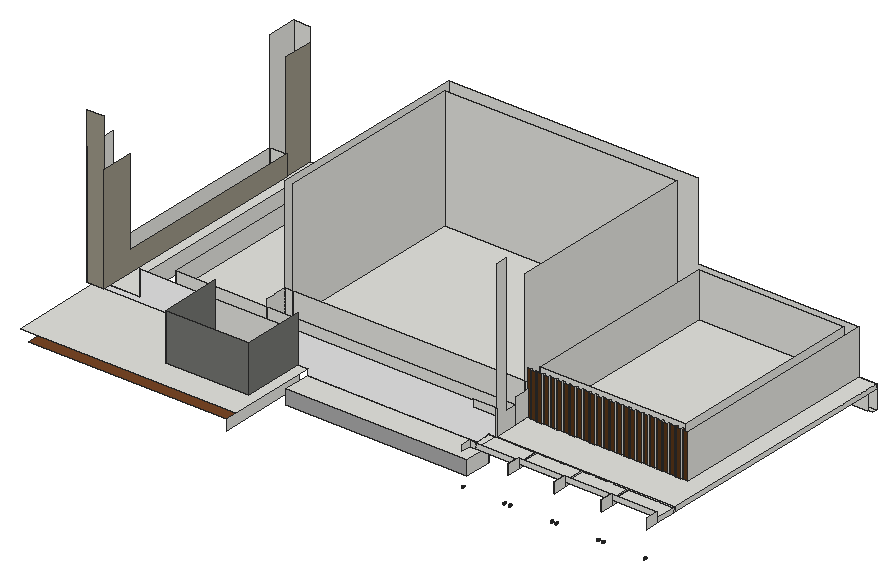
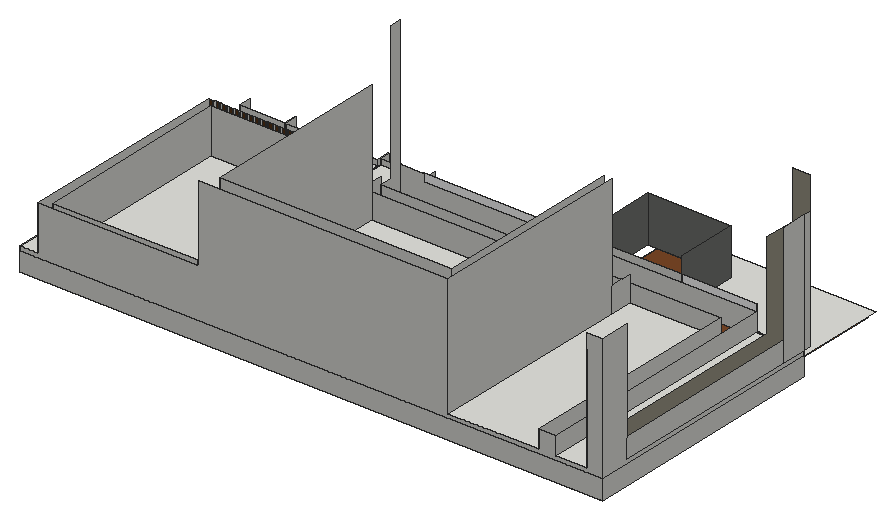
# SketchUp Ruby script. Lengths in inches.
U = 1.inch
M = Sketchup.active_model
def pt(a) = Geom::Point3d.new(a.map { |v| v * U })
def face(e, loops, mat)
  f = e.add_face(loops[0].map { |a| pt(a) })
  loops[1..].each { |l| e.add_face(l.map { |a| pt(a) }).erase! }
  f.material = f.back_material = mat if mat
  f
end
# faces: each face lists its corners as indices into pts; further lists are holes
def faces(e, pts, list, mat = nil) = list.each { |f| face(e, (f[0].is_a?(Array) ? f : [f]).map { |l| l.map { |i| pts[i] } }, mat) }
# xy, xz, yz: faces in a plane at the given z, y or x. An outline is a flat list of corners, or four numbers for a rectangle; further outlines are holes
def ring(l) = l.size == 4 ? [[l[0], l[1]], [l[2], l[1]], [l[2], l[3]], [l[0], l[3]]] : l.each_slice(2).to_a
def flat(e, list, mat, &to3) = list.each { |f| face(e, (f[0].is_a?(Array) ? f : [f]).map { |l| ring(l).map { |u, v| to3.(u, v) } }, mat) }
def xy(e, z, list, mat = nil) = flat(e, list, mat) { |x, y| [x, y, z] }
def xz(e, y, list, mat = nil) = flat(e, list, mat) { |x, z| [x, y, z] }
def yz(e, x, list, mat = nil) = flat(e, list, mat) { |y, z| [x, y, z] }
def lines(e, pts, list) = list.each { |a, b| e.add_line(pt(pts[a]), pt(pts[b])) }
# prism: a flat outline (further loops are holes) pulled along v
def prism(e, loops, v, mat = nil)
  f = face(e, loops, mat); d = Geom::Vector3d.new(v.map { |x| x * U })
  f.pushpull(f.normal.samedirection?(d) ? d.length : -d.length)
end
def box(e, o, s, mat = nil) = prism(e, [[o, [o[0] + s[0], o[1], o[2]], [o[0] + s[0], o[1] + s[1], o[2]], [o[0], o[1] + s[1], o[2]]]], [0, 0, s[2]], mat)
def at(x, y, z, deg = 0) = Geom::Transformation.translation(pt([x, y, z])) * Geom::Transformation.rotation(ORIGIN, Z_AXIS, deg.degrees)
def axes(o, x, y, z) = Geom::Transformation.new([*x, 0, *y, 0, *z, 0, *pt(o).to_a, 1])
def part(name) = M.definitions.add(name)
# library, detail: a bought-in or finely detailed component or shape, given as its bounding box
def library(name, o, s) = part(name).tap { |d| box(d.entities, o, s) }
def detail(e, o, s) = box(e.add_group.entities, o, s)
def put(e, d, t, mat = nil) = e.add_instance(d, t).tap { |i| i.material = mat if mat }
def group(e, t, mat = nil) = e.add_group.tap { |g| g.transformation = t; g.material = mat if mat }.entities
root = M.entities
M.materials.add("[0030_OldLace]").color = [86, 53, 24]
M.materials.add("[0128_White]").color = [255, 255, 255]
M.materials.add("[Color M03]").color = [170, 170, 170]
M.materials.add("[Concrete Tile]").color = [155, 150, 134]
M.materials.add("[Metal Seamed]").color = [116, 117, 113]
M.materials.add("[Wood Veneer 01]").color = [120, 70, 37]
xy(root,95.79,[[2444.05,846.1,2544.33,851.0625]])
xy(root,99.26,[[2381.36,810.97,2608.61,845.35]],"[Wood Veneer 01]")
xy(root,101.375,[[2305.05,845.35,2370.42,846.1],[2112.0625,846.1,2112.0625,1160.85,2840.8125,1160.85,2840.8125,1155.13,2117.78,1155.13,2117.78,851.0625,2305.05,851.0625,2305.05,846.1],[2305.05,846.1,2370.42,851.0625]])
xy(root,101.78,[[2134.72,845.35,2259.6,851.0625]])
xy(root,114.25,[[2123,732.28,2370.42,845.35]],"[Wood Veneer 01]")
xy(root,117.26,[[2381.36,810.97,2608.61,845.35]])
xy(root,125.1875,[[2112.0625,732.28,2381.36,732.28,2381.36,845.35,2369.43,845.35,2369.43,767.72,2265.24,767.72,2265.24,845.35,2112.0625,845.35],[2112.0625,845.35,2381.36,846.1]])
xy(root,131.1875,[[2608.61,814.22,2609.07,844.47],[2609.07,814.22,2617.01,844.47],[2617.01,814.22,2666.66,844.47],[2667.6,817.6,2724.71,844.47],[2725.77,817.6,2782.76,844.47],
  [2784.08,817.6,2840.8125,844.47],[2112.0625,837.03,2132.8125,845.35],[2608.61,844.47,2609.07,845.35],[2609.07,844.47,2617.01,845.35],[2617.01,844.47,2840.8125,846.1],
  [2112.0625,845.35,2132.8125,846.1],[2132.8125,845.35,2170.98,846.1],[2608.61,845.35,2609.07,846.1],[2609.07,845.35,2617.01,846.1],[2112.0625,846.1,2132.8125,877.14],
  [2132.8125,846.1,2170.98,846.1,2170.98,1160.85,2132.1875,1160.85,2132.1875,1122.97,2132.8125,1122.97],[2617.01,846.1,2840.8125,846.1,2840.8125,1160.85,2818.39,1160.85,2818.39,893.65,2812.24,893.65,2812.24,895.71,2810.07,895.71,2810.07,893.65,2803.93,893.65,2803.93,895.71,2801.76,895.71,2801.76,894.34,2795.61,894.34,2795.61,895.71,2793.45,895.71,2793.45,894.34,2787.3,894.34,2787.3,895.71,2785.14,895.71,2785.14,894.34,2778.99,894.34,2778.99,895.71,2776.82,895.71,2776.82,894.34,2770.68,894.34,2770.68,895.71,2768.51,895.71,2768.51,894.34,2762.36,894.34,2762.36,895.71,2760.2,895.71,2760.2,894.34,2754.05,894.34,2754.05,895.71,2751.89,895.71,2751.89,894.34,2745.74,894.34,2745.74,895.71,2743.57,895.71,2743.57,894.34,2737.43,894.34,2737.43,895.71,2735.26,895.71,2735.26,894.34,2729.11,894.34,2729.11,895.71,2726.95,895.71,2726.95,894.34,2720.8,894.34,2720.8,895.71,2718.64,895.71,2718.64,894.34,2712.49,894.34,2712.49,895.71,2710.32,895.71,2710.32,894.34,2704.18,894.34,2704.18,895.71,2702.01,895.71,2702.01,894.34,2695.86,894.34,2695.86,895.71,2693.7,895.71,2693.7,894.34,2687.55,894.34,2687.55,895.71,2685.39,895.71,2685.39,894.34,2679.24,894.34,2679.24,895.71,2677.07,895.71,2677.07,894.34,2670.93,894.34,2670.93,895.71,2668.76,895.71,2668.76,894.34,2662.61,894.34,2662.61,895.71,2660.45,895.71,2660.45,894.34,2654.3,894.34,2654.3,895.71,2652.14,895.71,2652.14,894.34,2645.99,894.34,2645.99,895.71,2643.82,895.71,2643.82,894.34,2637.68,894.34,2637.68,895.71,2635.51,895.71,2635.51,894.34,2629.36,894.34,2629.36,895.71,2627.2,895.71,2627.2,894.34,2621.05,894.34,2621.05,895.71,2617.01,895.71],[2112.0625,877.14,2132.8125,1122.97],[2191.39,877.14,2305.05,1160.85],[2305.05,877.14,2617.01,905.7],
  [2625.48,904.18,2807.17,1152.375],[2314.43,905.7,2604.75,1143.26]])
xz(root,767.72,[[2265.24,125.1875,2369.43,183.3125]],"[Metal Seamed]")
xz(root,799.91,[[2611.43,91.63,2611.73,91.67,2612,91.78,2612.23,91.96,2612.41,92.19,2612.52,92.46,2612.56,92.75,2612.52,93.04,2612.41,93.32,2612.23,93.55,2612,93.73,2611.73,93.84,2611.43,93.88,2611.14,93.84,2610.87,93.73,2610.64,93.55,2610.46,93.32,2610.35,93.04,2610.31,92.75,2610.35,92.46,2610.46,92.19,2610.64,91.96,2610.87,91.78,2611.14,91.67],[2663.62,91.63,2663.91,91.67,2664.18,91.78,2664.42,91.96,2664.6,92.19,2664.71,92.46,2664.75,92.75,2664.71,93.04,2664.6,93.32,2664.42,93.55,2664.18,93.73,2663.91,93.84,2663.62,93.88,2663.33,93.84,2663.06,93.73,2662.83,93.55,2662.65,93.32,2662.53,93.04,2662.5,92.75,2662.53,92.46,2662.65,92.19,2662.83,91.96,2663.06,91.78,2663.33,91.67],[2670.42,91.63,2670.71,91.67,2670.98,91.78,2671.22,91.96,2671.4,92.19,2671.51,92.46,2671.55,92.75,2671.51,93.04,2671.4,93.32,2671.22,93.55,2670.98,93.73,2670.71,93.84,2670.42,93.88,2670.13,93.84,2669.86,93.73,2669.625,93.55,2669.45,93.32,2669.34,93.04,2669.3,92.75,2669.34,92.46,2669.45,92.19,2669.625,91.96,2669.86,91.78,2670.13,91.67],[2722.61,91.63,2722.9,91.67,2723.17,91.78,2723.41,91.96,2723.58,92.19,2723.7,92.46,2723.73,92.75,2723.7,93.04,2723.58,93.32,2723.41,93.55,2723.17,93.73,2722.9,93.84,2722.61,93.88,2722.32,93.84,2722.05,93.73,2721.8125,93.55,2721.64,93.32,2721.52,93.04,2721.48,92.75,2721.52,92.46,2721.64,92.19,2721.8125,91.96,2722.05,91.78,2722.32,91.67],[2728.6,91.63,2728.89,91.67,2729.16,91.78,2729.39,91.96,2729.57,92.19,2729.68,92.46,2729.72,92.75,2729.68,93.04,2729.57,93.32,2729.39,93.55,2729.16,93.73,2728.89,93.84,2728.6,93.88,2728.31,93.84,2728.04,93.73,2727.8,93.55,2727.625,93.32,2727.51,93.04,2727.47,92.75,2727.51,92.46,2727.625,92.19,2727.8,91.96,2728.04,91.78,2728.31,91.67],
  [2780.79,91.63,2781.08,91.67,2781.35,91.78,2781.58,91.96,2781.76,92.19,2781.87,92.46,2781.91,92.75,2781.87,93.04,2781.76,93.32,2781.58,93.55,2781.35,93.73,2781.08,93.84,2780.79,93.88,2780.49,93.84,2780.22,93.73,2779.99,93.55,2779.8125,93.32,2779.7,93.04,2779.66,92.75,2779.7,92.46,2779.8125,92.19,2779.99,91.96,2780.22,91.78,2780.49,91.67],[2786.9,91.63,2787.19,91.67,2787.46,91.78,2787.69,91.96,2787.87,92.19,2787.99,92.46,2788.02,92.75,2787.99,93.04,2787.87,93.32,2787.69,93.55,2787.46,93.73,2787.19,93.84,2786.9,93.88,2786.61,93.84,2786.34,93.73,2786.1,93.55,2785.92,93.32,2785.8125,93.04,2785.77,92.75,2785.8125,92.46,2785.92,92.19,2786.1,91.96,2786.34,91.78,2786.61,91.67],[2839.09,91.63,2839.38,91.67,2839.65,91.78,2839.88,91.96,2840.06,92.19,2840.17,92.46,2840.21,92.75,2840.17,93.04,2840.06,93.32,2839.88,93.55,2839.65,93.73,2839.38,93.84,2839.09,93.88,2838.8,93.84,2838.52,93.73,2838.29,93.55,2838.11,93.32,2838,93.04,2837.96,92.75,2838,92.46,2838.11,92.19,2838.29,91.96,2838.52,91.78,2838.8,91.67]])
xz(root,810.97,[[2381.36,99.26,2608.61,117.26]],"[Color M03]")
xz(root,814.22,[[2608.61,131.1875,2617.01,138.0625],[2617.01,131.1875,2666.66,138.0625]])
xz(root,817.6,[[2667.6,131.1875,2724.71,138.0625],[2725.77,131.1875,2782.76,138.0625],[2784.08,131.1875,2840.8125,138.0625]])
xz(root,837.03,[[2112.0625,131.1875,2132.8125,324.5625]],"[Concrete Tile]")
xz(root,845.35,[[2381.36,99.26,2608.61,117.26],[2265.24,125.1875,2369.43,162.75]])
xz(root,845.35,[[2381.36,117.26,2608.61,117.26,2608.61,131.1875,2617.01,131.1875,2617.01,154.75,2587.8,154.75,2587.8,162.75,2369.43,162.75,2369.43,125.1875,2381.36,125.1875],[2112.0625,125.1875,2265.24,125.1875,2265.24,162.75,2170.98,162.75,2170.98,131.1875,2112.0625,131.1875]],"[0128_White]")
xz(root,846.1,[[2112.0625,125.1875,2112.0625,131.1875,2170.98,131.1875,2170.98,153.5625,2587.8,153.5625,2587.8,163,2617.01,163,2617.01,131.1875,2608.61,131.1875,2608.61,125.1875]])
xz(root,851.0625,[[2134.72,101.375,2259.6,101.78]])
xz(root,877.14,[[2191.39,131.1875,2305.05,153.5625],[2305.05,131.1875,2617.01,153.5625]])
xz(root,893.65,[[2803.93,131.1875,2810.07,186.75],[2812.24,131.1875,2818.39,186.75]],"[0030_OldLace]")
xz(root,894.34,[[2621.05,131.1875,2627.2,186.75],[2629.36,131.1875,2635.51,186.75],[2637.68,131.1875,2643.82,186.75],[2645.99,131.1875,2652.14,186.75],[2654.3,131.1875,2660.45,186.75],
  [2662.61,131.1875,2668.76,186.75],[2670.93,131.1875,2677.07,186.75],[2679.24,131.1875,2685.39,186.75],[2687.55,131.1875,2693.7,186.75],[2695.86,131.1875,2702.01,186.75],
  [2704.18,131.1875,2710.32,186.75],[2712.49,131.1875,2718.64,186.75],[2720.8,131.1875,2726.95,186.75],[2729.11,131.1875,2735.26,186.75],[2737.43,131.1875,2743.57,186.75],
  [2745.74,131.1875,2751.89,186.75],[2754.05,131.1875,2760.2,186.75],[2762.36,131.1875,2768.51,186.75],[2770.68,131.1875,2776.82,186.75],[2778.99,131.1875,2785.14,186.75],
  [2787.3,131.1875,2793.45,186.75],[2795.61,131.1875,2801.76,186.75]],"[0030_OldLace]")
xz(root,895.71,[[2617.01,131.1875,2621.05,186.75],[2627.2,131.1875,2629.36,186.75],[2635.51,131.1875,2637.68,186.75],[2643.82,131.1875,2645.99,186.75],[2652.14,131.1875,2654.3,186.75],
  [2660.45,131.1875,2662.61,186.75],[2668.76,131.1875,2670.93,186.75],[2677.07,131.1875,2679.24,186.75],[2685.39,131.1875,2687.55,186.75],[2693.7,131.1875,2695.86,186.75],
  [2702.01,131.1875,2704.18,186.75],[2710.32,131.1875,2712.49,186.75],[2718.64,131.1875,2720.8,186.75],[2726.95,131.1875,2729.11,186.75],[2735.26,131.1875,2737.43,186.75],
  [2743.57,131.1875,2745.74,186.75],[2751.89,131.1875,2754.05,186.75],[2760.2,131.1875,2762.36,186.75],[2768.51,131.1875,2770.68,186.75],[2776.82,131.1875,2778.99,186.75],
  [2785.14,131.1875,2787.3,186.75],[2793.45,131.1875,2795.61,186.75],[2801.76,131.1875,2803.93,186.75],[2810.07,131.1875,2812.24,186.75]],"[0030_OldLace]")
xz(root,904.18,[[2625.48,131.1875,2807.17,186.75]])
xz(root,905.7,[[2305.05,131.1875,2314.43,162.75],[2314.43,131.1875,2604.75,162.75],[2604.75,131.1875,2617.01,162.75]])
xz(root,1122.97,[[2112.0625,131.1875,2132.1875,156.5],[2132.1875,131.1875,2132.8125,156.5]])
xz(root,1143.26,[[2314.43,131.1875,2604.75,282.75]])
xz(root,1152.375,[[2625.48,131.1875,2807.17,186.75]])
xz(root,1155.13,[[2117.78,101.375,2835.1,125.1875]])
xz(root,1160.85,[[2112.0625,101.375,2840.8125,125.1875],[2112.0625,125.1875,2112.0625,282.75,2132.1875,282.75,2132.1875,131.1875,2170.98,131.1875,2170.98,153.5625,2191.39,153.5625,2191.39,131.1875,2305.05,131.1875,2305.05,282.75,2617.01,282.75,2617.01,186.75,2818.39,186.75,2818.39,131.1875,2840.8125,131.1875,2840.8125,125.1875]])
yz(root,2112.0625,[[846.1,101.375,1160.85,125.1875],[845.35,125.1875,846.1,131.1875],[846.1,125.1875,846.1,131.1875,1122.97,131.1875,1122.97,282.75,1160.85,282.75,1160.85,125.1875],[837.03,131.1875,845.35,282.75],[845.35,131.1875,877.14,282.75],
  [877.14,131.1875,1122.97,156.5]])
yz(root,2117.78,[[851.0625,101.375,1155.13,125.1875]])
yz(root,2132.1875,[[1122.97,131.1875,1160.85,264.75]],"[Concrete Tile]")
yz(root,2132.8125,[[837.03,131.1875,1122.97,131.1875,1122.97,156.5,877.14,156.5,877.14,264.75,837.03,264.75]],"[Concrete Tile]")
yz(root,2170.98,[[845.35,131.1875,846.1,162.75],[846.1,131.1875,1160.85,153.5625]])
yz(root,2191.39,[[877.14,131.1875,1160.85,153.5625]])
yz(root,2265.24,[[767.72,125.1875,845.35,183.3125]],"[Metal Seamed]")
yz(root,2305.05,[[877.14,131.1875,877.14,162.125,888.95,162.125,888.95,162.75,905.7,162.75,905.7,131.1875],[905.7,131.1875,1160.85,282.75]])
yz(root,2314.43,[[905.7,131.1875,1143.26,282.75]])
yz(root,2369.43,[[767.72,125.1875,845.35,183.3125]],"[Metal Seamed]")
yz(root,2370.42,[[732.28,101.375,845.35,114.25]])
yz(root,2604.75,[[905.7,131.1875,1143.26,282.75]])
yz(root,2608.61,[[810.97,99.26,844.47,117.26],[844.47,99.26,845.35,117.26],[844.47,117.26,845.35,125.1875],[844.47,125.1875,845.35,131.1875],[845.35,125.1875,846.1,131.1875],
  [801.78,131.1875,814.22,138.0625]])
yz(root,2617.01,[[845.35,131.1875,846.1,163],[846.1,131.1875,877.14,131.1875,877.14,153.5625,861.24,153.5625,861.24,324.5625,846.1,324.5625],[877.14,131.1875,895.71,131.1875,895.71,162.75,890.39,162.75,890.39,162.125,877.14,162.125],[895.71,131.1875,905.7,162.75]])
yz(root,2621.05,[[894.34,131.1875,895.71,186.75]])
yz(root,2625.48,[[904.18,131.1875,905.7,186.75],[905.7,131.1875,1152.375,186.75]])
yz(root,2627.2,[[894.34,131.1875,895.71,186.75]])
yz(root,2629.36,[[894.34,131.1875,895.71,186.75]])
yz(root,2635.51,[[894.34,131.1875,895.71,186.75]])
yz(root,2637.68,[[894.34,131.1875,895.71,186.75]])
yz(root,2643.82,[[894.34,131.1875,895.71,186.75]])
yz(root,2645.99,[[894.34,131.1875,895.71,186.75]])
yz(root,2652.14,[[894.34,131.1875,895.71,186.75]])
yz(root,2654.3,[[894.34,131.1875,895.71,186.75]])
yz(root,2660.45,[[894.34,131.1875,895.71,186.75]])
yz(root,2662.61,[[894.34,131.1875,895.71,186.75]])
yz(root,2666.66,[[801.78,125.1875,814.22,138.0625],[814.22,125.1875,844.47,131.1875]])
yz(root,2667.6,[[801.78,125.1875,817.6,138.0625],[817.6,125.1875,844.47,131.1875]])
yz(root,2668.76,[[894.34,131.1875,895.71,186.75]])
yz(root,2670.93,[[894.34,131.1875,895.71,186.75]])
yz(root,2677.07,[[894.34,131.1875,895.71,186.75]])
yz(root,2679.24,[[894.34,131.1875,895.71,186.75]])
yz(root,2685.39,[[894.34,131.1875,895.71,186.75]])
yz(root,2687.55,[[894.34,131.1875,895.71,186.75]])
yz(root,2693.7,[[894.34,131.1875,895.71,186.75]])
yz(root,2695.86,[[894.34,131.1875,895.71,186.75]])
yz(root,2702.01,[[894.34,131.1875,895.71,186.75]])
yz(root,2704.18,[[894.34,131.1875,895.71,186.75]])
yz(root,2710.32,[[894.34,131.1875,895.71,186.75]])
yz(root,2712.49,[[894.34,131.1875,895.71,186.75]])
yz(root,2718.64,[[894.34,131.1875,895.71,186.75]])
yz(root,2720.8,[[894.34,131.1875,895.71,186.75]])
yz(root,2724.71,[[801.78,125.1875,817.6,138.0625],[817.6,125.1875,844.47,131.1875]])
yz(root,2725.77,[[801.78,125.1875,817.6,138.0625],[817.6,125.1875,844.47,131.1875]])
yz(root,2726.95,[[894.34,131.1875,895.71,186.75]])
yz(root,2729.11,[[894.34,131.1875,895.71,186.75]])
yz(root,2735.26,[[894.34,131.1875,895.71,186.75]])
yz(root,2737.43,[[894.34,131.1875,895.71,186.75]])
yz(root,2743.57,[[894.34,131.1875,895.71,186.75]])
yz(root,2745.74,[[894.34,131.1875,895.71,186.75]])
yz(root,2751.89,[[894.34,131.1875,895.71,186.75]])
yz(root,2754.05,[[894.34,131.1875,895.71,186.75]])
yz(root,2760.2,[[894.34,131.1875,895.71,186.75]])
yz(root,2762.36,[[894.34,131.1875,895.71,186.75]])
yz(root,2768.51,[[894.34,131.1875,895.71,186.75]])
yz(root,2770.68,[[894.34,131.1875,895.71,186.75]])
yz(root,2776.82,[[894.34,131.1875,895.71,186.75]])
yz(root,2778.99,[[894.34,131.1875,895.71,186.75]])
yz(root,2782.76,[[801.78,125.1875,817.6,138.0625],[817.6,125.1875,844.47,131.1875]])
yz(root,2784.08,[[801.78,125.1875,817.6,138.0625],[817.6,125.1875,844.47,131.1875]])
yz(root,2785.14,[[894.34,131.1875,895.71,186.75]])
yz(root,2787.3,[[894.34,131.1875,895.71,186.75]])
yz(root,2793.45,[[894.34,131.1875,895.71,186.75]])
yz(root,2795.61,[[894.34,131.1875,895.71,186.75]],"[0030_OldLace]")
yz(root,2801.76,[[894.34,131.1875,895.71,186.75]])
yz(root,2803.93,[[893.65,131.1875,895.71,186.75]],"[0030_OldLace]")
yz(root,2807.17,[[904.18,131.1875,1152.375,186.75]])
yz(root,2810.07,[[893.65,131.1875,895.71,186.75]])
yz(root,2812.24,[[893.65,131.1875,895.71,186.75]],"[0030_OldLace]")
yz(root,2818.39,[[893.65,131.1875,1160.85,186.75]])
yz(root,2840.8125,[[801.78,125.1875,817.6,138.0625],[817.6,125.1875,844.47,131.1875],[844.47,125.1875,846.1,131.1875],[846.1,125.1875,1160.85,131.1875]])
p = [[2611.14,801.78,91.67],[2611.43,801.78,91.63],[2611.43,799.91,91.63],[2611.14,799.91,91.67],[2611.73,801.78,91.67],[2611.73,799.91,91.67],
  [2663.33,801.78,91.67],[2663.62,801.78,91.63],[2663.62,799.91,91.63],[2663.33,799.91,91.67],[2663.91,801.78,91.67],[2663.91,799.91,91.67],
  [2670.13,801.78,91.67],[2670.42,801.78,91.63],[2670.42,799.91,91.63],[2670.13,799.91,91.67],[2670.71,801.78,91.67],[2670.71,799.91,91.67],
  [2722.32,801.78,91.67],[2722.61,801.78,91.63],[2722.61,799.91,91.63],[2722.32,799.91,91.67],[2722.9,801.78,91.67],[2722.9,799.91,91.67],
  [2728.31,801.78,91.67],[2728.6,801.78,91.63],[2728.6,799.91,91.63],[2728.31,799.91,91.67],[2728.89,801.78,91.67],[2728.89,799.91,91.67],
  [2780.49,801.78,91.67],[2780.79,801.78,91.63],[2780.79,799.91,91.63],[2780.49,799.91,91.67],[2781.08,801.78,91.67],[2781.08,799.91,91.67],
  [2786.61,801.78,91.67],[2786.9,801.78,91.63],[2786.9,799.91,91.63],[2786.61,799.91,91.67],[2787.19,801.78,91.67],[2787.19,799.91,91.67],
  [2838.8,801.78,91.67],[2839.09,801.78,91.63],[2839.09,799.91,91.63],[2838.8,799.91,91.67],[2839.38,801.78,91.67],[2839.38,799.91,91.67],
  [2610.87,801.78,91.78],[2610.87,799.91,91.78],[2612,801.78,91.78],[2612,799.91,91.78],[2663.06,801.78,91.78],[2663.06,799.91,91.78],
  [2664.18,801.78,91.78],[2664.18,799.91,91.78],[2669.86,801.78,91.78],[2669.86,799.91,91.78],[2670.98,801.78,91.78],[2670.98,799.91,91.78],
  [2722.05,801.78,91.78],[2722.05,799.91,91.78],[2723.17,801.78,91.78],[2723.17,799.91,91.78],[2728.04,801.78,91.78],[2728.04,799.91,91.78],
  [2729.16,801.78,91.78],[2729.16,799.91,91.78],[2780.22,801.78,91.78],[2780.22,799.91,91.78],[2781.35,801.78,91.78],[2781.35,799.91,91.78],
  [2786.34,801.78,91.78],[2786.34,799.91,91.78],[2787.46,801.78,91.78],[2787.46,799.91,91.78],[2838.52,801.78,91.78],[2838.52,799.91,91.78],
  [2839.65,801.78,91.78],[2839.65,799.91,91.78],[2610.64,801.78,91.96],[2610.64,799.91,91.96],[2612.23,801.78,91.96],[2612.23,799.91,91.96],
  [2662.83,801.78,91.96],[2662.83,799.91,91.96],[2664.42,801.78,91.96],[2664.42,799.91,91.96],[2669.625,801.78,91.96],[2669.625,799.91,91.96],
  [2671.22,801.78,91.96],[2671.22,799.91,91.96],[2721.8125,801.78,91.96],[2721.8125,799.91,91.96],[2723.41,801.78,91.96],[2723.41,799.91,91.96],
  [2727.8,801.78,91.96],[2727.8,799.91,91.96],[2729.39,801.78,91.96],[2729.39,799.91,91.96],[2779.99,801.78,91.96],[2779.99,799.91,91.96],
  [2781.58,801.78,91.96],[2781.58,799.91,91.96],[2786.1,801.78,91.96],[2786.1,799.91,91.96],[2787.69,801.78,91.96],[2787.69,799.91,91.96],
  [2838.29,801.78,91.96],[2838.29,799.91,91.96],[2839.88,801.78,91.96],[2839.88,799.91,91.96],[2610.46,801.78,92.19],[2610.46,799.91,92.19],
  [2612.41,801.78,92.19],[2612.41,799.91,92.19],[2662.65,801.78,92.19],[2662.65,799.91,92.19],[2664.6,801.78,92.19],[2664.6,799.91,92.19],
  [2669.45,801.78,92.19],[2669.45,799.91,92.19],[2671.4,801.78,92.19],[2671.4,799.91,92.19],[2721.64,801.78,92.19],[2721.64,799.91,92.19],
  [2723.58,801.78,92.19],[2723.58,799.91,92.19],[2727.625,801.78,92.19],[2727.625,799.91,92.19],[2729.57,801.78,92.19],[2729.57,799.91,92.19],
  [2779.8125,801.78,92.19],[2779.8125,799.91,92.19],[2781.76,801.78,92.19],[2781.76,799.91,92.19],[2785.92,801.78,92.19],[2785.92,799.91,92.19],
  [2787.87,801.78,92.19],[2787.87,799.91,92.19],[2838.11,801.78,92.19],[2838.11,799.91,92.19],[2840.06,801.78,92.19],[2840.06,799.91,92.19],
  [2610.35,801.78,92.46],[2610.35,799.91,92.46],[2612.52,801.78,92.46],[2612.52,799.91,92.46],[2662.53,801.78,92.46],[2662.53,799.91,92.46],
  [2664.71,801.78,92.46],[2664.71,799.91,92.46],[2669.34,801.78,92.46],[2669.34,799.91,92.46],[2671.51,801.78,92.46],[2671.51,799.91,92.46],
  [2721.52,801.78,92.46],[2721.52,799.91,92.46],[2723.7,801.78,92.46],[2723.7,799.91,92.46],[2727.51,801.78,92.46],[2727.51,799.91,92.46],
  [2729.68,801.78,92.46],[2729.68,799.91,92.46],[2779.7,801.78,92.46],[2779.7,799.91,92.46],[2781.87,801.78,92.46],[2781.87,799.91,92.46],
  [2785.8125,801.78,92.46],[2785.8125,799.91,92.46],[2787.99,801.78,92.46],[2787.99,799.91,92.46],[2838,801.78,92.46],[2838,799.91,92.46],
  [2840.17,801.78,92.46],[2840.17,799.91,92.46],[2610.31,801.78,92.75],[2610.31,799.91,92.75],[2612.56,801.78,92.75],[2612.56,799.91,92.75],
  [2662.5,801.78,92.75],[2662.5,799.91,92.75],[2664.75,801.78,92.75],[2664.75,799.91,92.75],[2669.3,801.78,92.75],[2669.3,799.91,92.75],
  [2671.55,801.78,92.75],[2671.55,799.91,92.75],[2721.48,801.78,92.75],[2721.48,799.91,92.75],[2723.73,801.78,92.75],[2723.73,799.91,92.75],
  [2727.47,801.78,92.75],[2727.47,799.91,92.75],[2729.72,801.78,92.75],[2729.72,799.91,92.75],[2779.66,801.78,92.75],[2779.66,799.91,92.75],
  [2781.91,801.78,92.75],[2781.91,799.91,92.75],[2785.77,801.78,92.75],[2785.77,799.91,92.75],[2788.02,801.78,92.75],[2788.02,799.91,92.75],
  [2837.96,801.78,92.75],[2837.96,799.91,92.75],[2840.21,801.78,92.75],[2840.21,799.91,92.75],[2610.35,801.78,93.04],[2610.35,799.91,93.04],
  [2612.52,801.78,93.04],[2612.52,799.91,93.04],[2662.53,801.78,93.04],[2662.53,799.91,93.04],[2664.71,801.78,93.04],[2664.71,799.91,93.04],
  [2669.34,801.78,93.04],[2669.34,799.91,93.04],[2671.51,801.78,93.04],[2671.51,799.91,93.04],[2721.52,801.78,93.04],[2721.52,799.91,93.04],
  [2723.7,801.78,93.04],[2723.7,799.91,93.04],[2727.51,801.78,93.04],[2727.51,799.91,93.04],[2729.68,801.78,93.04],[2729.68,799.91,93.04],
  [2779.7,801.78,93.04],[2779.7,799.91,93.04],[2781.87,801.78,93.04],[2781.87,799.91,93.04],[2785.8125,801.78,93.04],[2785.8125,799.91,93.04],
  [2787.99,801.78,93.04],[2787.99,799.91,93.04],[2838,801.78,93.04],[2838,799.91,93.04],[2840.17,801.78,93.04],[2840.17,799.91,93.04],
  [2610.46,801.78,93.32],[2610.46,799.91,93.32],[2612.41,801.78,93.32],[2612.41,799.91,93.32],[2662.65,801.78,93.32],[2662.65,799.91,93.32],
  [2664.6,801.78,93.32],[2664.6,799.91,93.32],[2669.45,801.78,93.32],[2669.45,799.91,93.32],[2671.4,801.78,93.32],[2671.4,799.91,93.32],
  [2721.64,801.78,93.32],[2721.64,799.91,93.32],[2723.58,801.78,93.32],[2723.58,799.91,93.32],[2727.625,801.78,93.32],[2727.625,799.91,93.32],
  [2729.57,801.78,93.32],[2729.57,799.91,93.32],[2779.8125,801.78,93.32],[2779.8125,799.91,93.32],[2781.76,801.78,93.32],[2781.76,799.91,93.32],
  [2785.92,801.78,93.32],[2785.92,799.91,93.32],[2787.87,801.78,93.32],[2787.87,799.91,93.32],[2838.11,801.78,93.32],[2838.11,799.91,93.32],
  [2840.06,801.78,93.32],[2840.06,799.91,93.32],[2610.64,801.78,93.55],[2610.64,799.91,93.55],[2612.23,801.78,93.55],[2612.23,799.91,93.55],
  [2662.83,801.78,93.55],[2662.83,799.91,93.55],[2664.42,801.78,93.55],[2664.42,799.91,93.55],[2669.625,801.78,93.55],[2669.625,799.91,93.55],
  [2671.22,801.78,93.55],[2671.22,799.91,93.55],[2721.8125,801.78,93.55],[2721.8125,799.91,93.55],[2723.41,801.78,93.55],[2723.41,799.91,93.55],
  [2727.8,801.78,93.55],[2727.8,799.91,93.55],[2729.39,801.78,93.55],[2729.39,799.91,93.55],[2779.99,801.78,93.55],[2779.99,799.91,93.55],
  [2781.58,801.78,93.55],[2781.58,799.91,93.55],[2786.1,801.78,93.55],[2786.1,799.91,93.55],[2787.69,801.78,93.55],[2787.69,799.91,93.55],
  [2838.29,801.78,93.55],[2838.29,799.91,93.55],[2839.88,801.78,93.55],[2839.88,799.91,93.55],[2610.87,801.78,93.73],[2610.87,799.91,93.73],
  [2612,801.78,93.73],[2612,799.91,93.73],[2663.06,801.78,93.73],[2663.06,799.91,93.73],[2664.18,801.78,93.73],[2664.18,799.91,93.73],
  [2669.86,801.78,93.73],[2669.86,799.91,93.73],[2670.98,801.78,93.73],[2670.98,799.91,93.73],[2722.05,801.78,93.73],[2722.05,799.91,93.73],
  [2723.17,801.78,93.73],[2723.17,799.91,93.73],[2728.04,801.78,93.73],[2728.04,799.91,93.73],[2729.16,801.78,93.73],[2729.16,799.91,93.73],
  [2780.22,801.78,93.73],[2780.22,799.91,93.73],[2781.35,801.78,93.73],[2781.35,799.91,93.73],[2786.34,801.78,93.73],[2786.34,799.91,93.73],
  [2787.46,801.78,93.73],[2787.46,799.91,93.73],[2838.52,801.78,93.73],[2838.52,799.91,93.73],[2839.65,801.78,93.73],[2839.65,799.91,93.73],
  [2611.14,801.78,93.84],[2611.14,799.91,93.84],[2611.73,801.78,93.84],[2611.73,799.91,93.84],[2663.33,801.78,93.84],[2663.33,799.91,93.84],
  [2663.91,801.78,93.84],[2663.91,799.91,93.84],[2670.13,801.78,93.84],[2670.13,799.91,93.84],[2670.71,801.78,93.84],[2670.71,799.91,93.84],
  [2722.32,801.78,93.84],[2722.32,799.91,93.84],[2722.9,801.78,93.84],[2722.9,799.91,93.84],[2728.31,801.78,93.84],[2728.31,799.91,93.84],
  [2728.89,801.78,93.84],[2728.89,799.91,93.84],[2780.49,801.78,93.84],[2780.49,799.91,93.84],[2781.08,801.78,93.84],[2781.08,799.91,93.84],
  [2786.61,801.78,93.84],[2786.61,799.91,93.84],[2787.19,801.78,93.84],[2787.19,799.91,93.84],[2838.8,801.78,93.84],[2838.8,799.91,93.84],
  [2839.38,801.78,93.84],[2839.38,799.91,93.84],[2611.43,801.78,93.88],[2611.43,799.91,93.88],[2663.62,801.78,93.88],[2663.62,799.91,93.88],
  [2670.42,801.78,93.88],[2670.42,799.91,93.88],[2722.61,801.78,93.88],[2722.61,799.91,93.88],[2728.6,801.78,93.88],[2728.6,799.91,93.88],
  [2780.79,801.78,93.88],[2780.79,799.91,93.88],[2786.9,801.78,93.88],[2786.9,799.91,93.88],[2839.09,801.78,93.88],[2839.09,799.91,93.88]]
faces(root,p,[[0,1,2,3],[1,4,5,2],[6,7,8,9],[7,10,11,8],[12,13,14,15],[13,16,17,14],[18,19,20,21],[19,22,23,20],
  [24,25,26,27],[25,28,29,26],[30,31,32,33],[31,34,35,32],[36,37,38,39],[37,40,41,38],[42,43,44,45],[43,46,47,44],
  [48,0,3,49],[4,50,51,5],[52,6,9,53],[10,54,55,11],[56,12,15,57],[16,58,59,17],[60,18,21,61],[22,62,63,23],
  [64,24,27,65],[28,66,67,29],[68,30,33,69],[34,70,71,35],[72,36,39,73],[40,74,75,41],[76,42,45,77],[46,78,79,47],
  [80,48,49,81],[50,82,83,51],[84,52,53,85],[54,86,87,55],[88,56,57,89],[58,90,91,59],[92,60,61,93],[62,94,95,63],
  [96,64,65,97],[66,98,99,67],[100,68,69,101],[70,102,103,71],[104,72,73,105],[74,106,107,75],[108,76,77,109],[78,110,111,79],
  [112,80,81,113],[82,114,115,83],[116,84,85,117],[86,118,119,87],[120,88,89,121],[90,122,123,91],[124,92,93,125],[94,126,127,95],
  [128,96,97,129],[98,130,131,99],[132,100,101,133],[102,134,135,103],[136,104,105,137],[106,138,139,107],[140,108,109,141],[110,142,143,111],
  [144,112,113,145],[114,146,147,115],[148,116,117,149],[118,150,151,119],[152,120,121,153],[122,154,155,123],[156,124,125,157],[126,158,159,127],
  [160,128,129,161],[130,162,163,131],[164,132,133,165],[134,166,167,135],[168,136,137,169],[138,170,171,139],[172,140,141,173],[142,174,175,143],
  [176,144,145,177],[146,178,179,147],[180,148,149,181],[150,182,183,151],[184,152,153,185],[154,186,187,155],[188,156,157,189],[158,190,191,159],
  [192,160,161,193],[162,194,195,163],[196,164,165,197],[166,198,199,167],[200,168,169,201],[170,202,203,171],[204,172,173,205],[174,206,207,175],
  [208,176,177,209],[178,210,211,179],[212,180,181,213],[182,214,215,183],[216,184,185,217],[186,218,219,187],[220,188,189,221],[190,222,223,191],
  [224,192,193,225],[194,226,227,195],[228,196,197,229],[198,230,231,199],[232,200,201,233],[202,234,235,203],[236,204,205,237],[206,238,239,207],
  [240,208,209,241],[210,242,243,211],[244,212,213,245],[214,246,247,215],[248,216,217,249],[218,250,251,219],[252,220,221,253],[222,254,255,223],
  [256,224,225,257],[226,258,259,227],[260,228,229,261],[230,262,263,231],[264,232,233,265],[234,266,267,235],[268,236,237,269],[238,270,271,239],
  [272,240,241,273],[242,274,275,243],[276,244,245,277],[246,278,279,247],[280,248,249,281],[250,282,283,251],[284,252,253,285],[254,286,287,255],
  [288,256,257,289],[258,290,291,259],[292,260,261,293],[262,294,295,263],[296,264,265,297],[266,298,299,267],[300,268,269,301],[270,302,303,271],
  [304,272,273,305],[274,306,307,275],[308,276,277,309],[278,310,311,279],[312,280,281,313],[282,314,315,283],[316,284,285,317],[286,318,319,287],
  [320,288,289,321],[290,322,323,291],[324,292,293,325],[294,326,327,295],[328,296,297,329],[298,330,331,299],[332,300,301,333],[302,334,335,303],
  [336,304,305,337],[306,338,339,307],[340,308,309,341],[310,342,343,311],[344,312,313,345],[314,346,347,315],[348,316,317,349],[318,350,351,319],
  [352,320,321,353],[322,354,355,323],[356,324,325,357],[326,358,359,327],[360,328,329,361],[330,362,363,331],[364,332,333,365],[334,366,367,335],
  [368,336,337,369],[338,368,369,339],[370,340,341,371],[342,370,371,343],[372,344,345,373],[346,372,373,347],[374,348,349,375],[350,374,375,351],
  [376,352,353,377],[354,376,377,355],[378,356,357,379],[358,378,379,359],[380,360,361,381],[362,380,381,363],[382,364,365,383],[366,382,383,367]])
